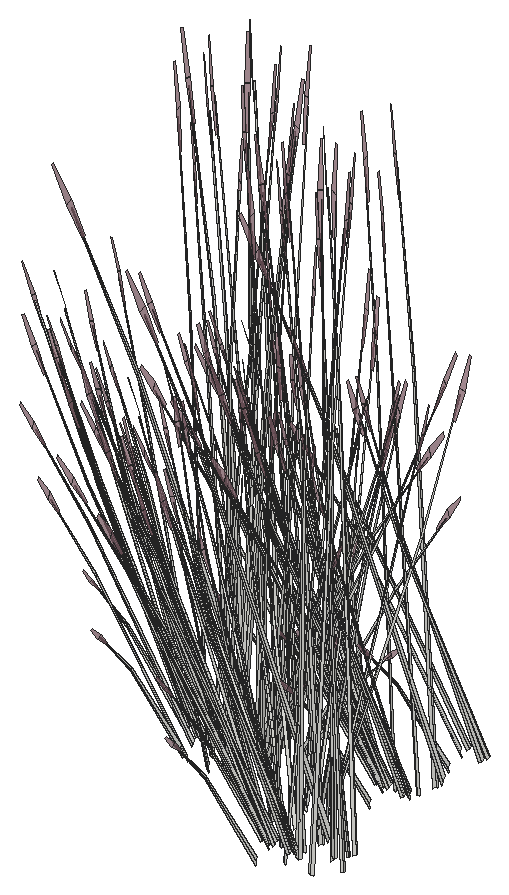
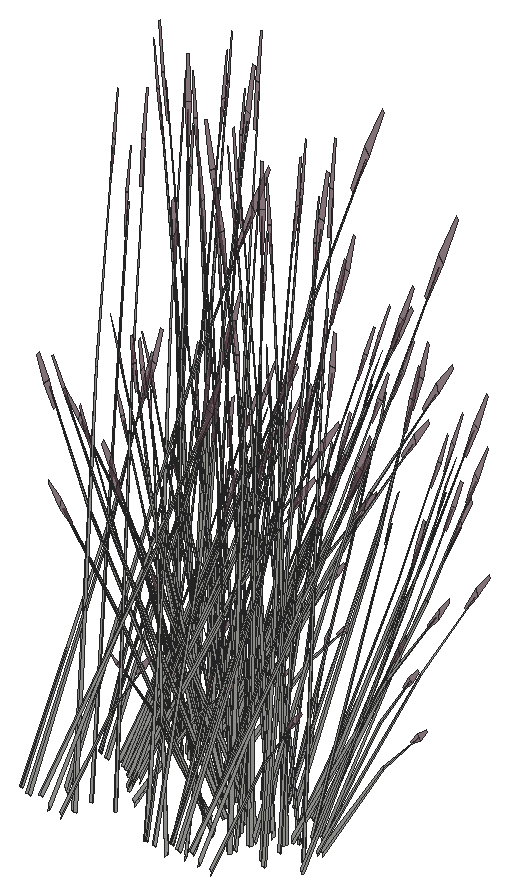
# SketchUp Ruby script. Lengths in inches.
U = 1.inch
M = Sketchup.active_model
def pt(a) = Geom::Point3d.new(a.map { |v| v * U })
def face(e, loops, mat)
  f = e.add_face(loops[0].map { |a| pt(a) })
  loops[1..].each { |l| e.add_face(l.map { |a| pt(a) }).erase! }
  f.material = f.back_material = mat if mat
  f
end
# faces: each face lists its corners as indices into pts; further lists are holes
def faces(e, pts, list, mat = nil) = list.each { |f| face(e, (f[0].is_a?(Array) ? f : [f]).map { |l| l.map { |i| pts[i] } }, mat) }
# xy, xz, yz: faces in a plane at the given z, y or x. An outline is a flat list of corners, or four numbers for a rectangle; further outlines are holes
def ring(l) = l.size == 4 ? [[l[0], l[1]], [l[2], l[1]], [l[2], l[3]], [l[0], l[3]]] : l.each_slice(2).to_a
def flat(e, list, mat, &to3) = list.each { |f| face(e, (f[0].is_a?(Array) ? f : [f]).map { |l| ring(l).map { |u, v| to3.(u, v) } }, mat) }
def xy(e, z, list, mat = nil) = flat(e, list, mat) { |x, y| [x, y, z] }
def xz(e, y, list, mat = nil) = flat(e, list, mat) { |x, z| [x, y, z] }
def yz(e, x, list, mat = nil) = flat(e, list, mat) { |y, z| [x, y, z] }
def lines(e, pts, list) = list.each { |a, b| e.add_line(pt(pts[a]), pt(pts[b])) }
# prism: a flat outline (further loops are holes) pulled along v
def prism(e, loops, v, mat = nil)
  f = face(e, loops, mat); d = Geom::Vector3d.new(v.map { |x| x * U })
  f.pushpull(f.normal.samedirection?(d) ? d.length : -d.length)
end
def box(e, o, s, mat = nil) = prism(e, [[o, [o[0] + s[0], o[1], o[2]], [o[0] + s[0], o[1] + s[1], o[2]], [o[0], o[1] + s[1], o[2]]]], [0, 0, s[2]], mat)
def at(x, y, z, deg = 0) = Geom::Transformation.translation(pt([x, y, z])) * Geom::Transformation.rotation(ORIGIN, Z_AXIS, deg.degrees)
def axes(o, x, y, z) = Geom::Transformation.new([*x, 0, *y, 0, *z, 0, *pt(o).to_a, 1])
def part(name) = M.definitions.add(name)
# library, detail: a bought-in or finely detailed component or shape, given as its bounding box
def library(name, o, s) = part(name).tap { |d| box(d.entities, o, s) }
def detail(e, o, s) = box(e.add_group.entities, o, s)
def put(e, d, t, mat = nil) = e.add_instance(d, t).tap { |i| i.material = mat if mat }
def group(e, t, mat = nil) = e.add_group.tap { |g| g.transformation = t; g.material = mat if mat }.entities
root = M.entities
M.materials.add("LightPink_Translucent").color = [144, 107, 117]
M.materials["LightPink_Translucent"].alpha = 0.75
c1 = part("blade")
p = [[2.15,0.21,22],[0,0.17,0],[0.09,0.45,0],[2.18,0.31,22],[2.29,0.31,22],[0.38,0.45,0],
  [2.48,0.24,33],[2.49,0.24,33],[2.48,0.22,33]]
faces(c1.entities,p,[[0,1,2,3],[4,5,2,3],[6,3,4,7],[8,0,3,6]])
c2 = part("seeds")
p = [[0.3,-0.1,1.38],[-0.01,-0.03,1.59],[-0.01,-0.03,0.03],[0.14,-0.07,-0.07],[0.29,-0.03,3],[0.15,0.01,3.11]]
faces(c2.entities,p,[[0,1,2,3],[1,0,4,5]],"LightPink_Translucent")
c3 = part("blade with seeds")
put(c3.entities,c1,at(0,0,0))
put(c3.entities,c2,axes([2.4,0.25,30.99],[1.5799,-0.05474,1.17369],[-0.12525,1.92788,0.29478],[-0.07173,-0.02425,1.56792]))
put(root,c3,axes([675.71,330.72,513.22],[0.14872,0.18332,1.42242],[-0.6872,0.15433,0.11501],[-0.15531,-0.28779,0.60807]))
put(root,c3,axes([677.54,330.86,514.13],[-0.31051,-0.46426,-0.58968],[0.63919,-0.25873,0.07116],[-0.07261,-0.22432,0.83415]))
put(root,c3,axes([677.6,330.46,513.76],[0.19614,-0.43908,-0.29394],[0.57222,0.12807,0.37948],[-0.05247,-0.17678,0.72609]))
put(root,c3,axes([677.31,330.76,513.89],[-0.63954,-0.14313,-0.42412],[0.21921,-0.49074,-0.32852],[-0.05864,-0.19758,0.81151]))
put(root,c3,axes([675.33,329.93,512.3],[0.33937,0.19872,0.95334],[-0.49424,0.11946,0.70045],[-0.10575,-0.15273,0.20998]))
put(root,c3,axes([676.14,330.99,514.13],[-0.55475,-0.27598,-0.58968],[0.39425,-0.48361,0.07116],[-0.20099,-0.16478,0.83415]))
put(root,c3,axes([675.95,330.62,513.76],[-0.10048,-0.4599,-0.29394],[0.5744,-0.12144,0.37948],[-0.15428,-0.13179,0.72609]))
put(root,c3,axes([674.72,331.29,513.22],[0.24166,0.09837,1.42242],[-0.50011,0.41269,0.11501],[-0.3117,-0.18617,0.60807]))
put(root,c3,axes([675.88,331,513.89],[-0.64198,0.13573,-0.42412],[-0.1123,-0.514,-0.32852],[-0.17243,-0.1473,0.81151]))
put(root,c3,axes([677.47,334.11,512.76],[0.56221,0.23024,1.25546],[-0.55078,0.49601,0.49647],[-0.2467,-0.29398,1.05249]))
put(root,c3,axes([674.62,331.43,513.76],[-0.37017,-0.35748,-0.29394],[0.42268,-0.3384,0.37948],[-0.21476,-0.05149,0.72609]))
put(root,c3,axes([675.01,331.67,514.13],[-0.65035,-0.01375,-0.58968],[0.04368,-0.5789,0.07116],[-0.27552,-0.06109,0.83415]))
put(root,c3,axes([674.8,331.79,513.89],[-0.47241,0.37822,-0.42412],[-0.41372,-0.39954,-0.32852],[-0.24002,-0.05755,0.81151]))
put(root,c3,axes([673.73,332.29,512.3],[0.41536,-0.04086,0.95334],[-0.26347,0.35999,0.70045],[-0.20525,-0.054,0.20998]))
put(root,c3,axes([676.67,332.62,512.26],[-0.70648,0.03525,0.37133],[-0.06389,-0.58508,-0.17871],[0.12647,-0.0593,1.19224]))
put(root,c3,axes([674.84,333.05,512.06],[0,0.57097,0.4121],[-0.72788,0,0],[0,-0.13004,1.30728]))
put(root,c3,axes([674.21,332.19,513.22],[0.26985,-0.01293,1.42242],[-0.17902,0.56047,0.11501],[-0.38456,-0.03467,0.60807]))
put(root,c3,axes([676.5,333.34,512.26],[-0.31565,0.51449,0.37133],[-0.65588,-0.24761,-0.17871],[0,-0.1186,1.19224]))
put(root,c3,axes([676.34,331.62,512.05],[-0.18794,0.56744,0.14643],[-0.68774,-0.16058,0.29122],[0.1188,-0.00276,1.33138]))
put(root,c3,axes([676.27,334.54,512.05],[0.6991,-0.15154,0.14643],[0.17263,0.56398,0.29122],[-0.06235,-0.08217,1.33138]))
put(root,c3,axes([673.97,332.67,513.76],[-0.54068,-0.15928,-0.29394],[0.1577,-0.46469,0.37948],[-0.21769,0.04261,0.72609]))
put(root,c3,axes([678.42,331.65,512.05],[-0.6991,0.15154,0.14643],[-0.17263,-0.56398,0.29122],[0.06235,0.08217,1.33138]))
put(root,c3,axes([666.76,337.92,512.15],[-0.18493,0.11557,1.18691],[-0.55384,-0.20228,-0.25526],[0.10266,-0.25157,0.50747]))
put(root,c3,axes([665.92,338.32,514.13],[-0.31051,-0.46426,-0.58968],[0.63919,-0.25873,0.07116],[-0.07261,-0.22432,0.83415]))
put(root,c3,axes([663.9,337.7,512.15],[-0.0394,0.18678,1.18691],[-0.57594,0.15636,-0.25526],[-0.13463,-0.24142,0.50747]))
put(root,c3,axes([678.35,334.57,512.05],[0.18794,-0.56744,0.14643],[0.68774,0.16058,0.29122],[-0.1188,0.00276,1.33138]))
put(root,c3,axes([667.21,338.77,514.13],[0.01693,-0.52814,-0.58968],[0.71285,0.03547,0.07116],[0.07523,-0.22375,0.83415]))
put(root,c3,axes([675.62,332.59,512.77],[0.18493,-0.0826,1.46963],[0.06377,0.5767,0.11501],[-0.40056,0.07652,0.52526]))
put(root,c3,axes([679.43,333.125,512.05],[-0.51116,-0.4159,0.14643],[0.51512,-0.4034,0.29122],[-0.05645,0.08494,1.33138]))
put(root,c3,axes([665.98,337.93,513.76],[0.19614,-0.43908,-0.29394],[0.57222,0.12807,0.37948],[-0.05247,-0.17678,0.72609]))
put(root,c3,axes([666.41,338.51,513.22],[-0.12114,0.19625,1.42242],[-0.50818,-0.40613,0.11501],[0.22925,-0.25313,0.60807]))
put(root,c3,axes([676.04,334.83,512.06],[0.60889,0.28548,0.4121],[-0.36394,0.51192,0],[-0.13868,-0.06502,1.30728]))
put(root,c3,axes([665.68,338.23,513.89],[-0.63954,-0.14313,-0.42412],[0.21921,-0.49074,-0.32852],[-0.05864,-0.19758,0.81151]))
put(root,c3,axes([666.08,337,512.3],[0.08346,0.33295,0.95334],[-0.46298,-0.1844,0.70045],[0.04982,-0.17048,0.20998]))
put(root,c3,axes([667.07,338.6,513.89],[-0.46573,-0.38364,-0.42412],[0.49199,-0.33598,-0.32852],[0.07086,-0.19492,0.81151]))
put(root,c3,axes([674.34,332.91,513.89],[-0.17625,0.51936,-0.42412],[-0.60429,-0.17802,-0.32852],[-0.2433,0.04762,0.81151]))
put(root,c3,axes([678.02,333.57,512.26],[0.70648,-0.03525,0.37133],[0.06389,0.58508,-0.17871],[-0.12647,0.0593,1.19224]))
put(root,c3,axes([667.5,338.46,513.76],[0.4402,-0.30062,-0.29394],[0.41671,0.34326,0.37948],[0.0634,-0.1744,0.72609]))
put(root,c3,axes([663.7,337.4,512.3],[0.33937,0.19872,0.95334],[-0.49424,0.11946,0.70045],[-0.10575,-0.15273,0.20998]))
put(root,c3,axes([664.52,338.45,514.13],[-0.55475,-0.27598,-0.58968],[0.39425,-0.48361,0.07116],[-0.20099,-0.16478,0.83415]))
put(root,c3,axes([664.33,338.09,513.76],[-0.10048,-0.4599,-0.29394],[0.5744,-0.12144,0.37948],[-0.15428,-0.13179,0.72609]))
put(root,c3,axes([674.32,333.18,513.22],[0.22574,-0.12077,1.42242],[0.19004,0.55807,0.11501],[-0.35439,0.12613,0.60807]))
put(root,c3,axes([676.7,340.4,513.22],[0.14872,0.18332,1.42242],[-0.6872,0.15433,0.11501],[-0.15531,-0.28779,0.60807]))
put(root,c3,axes([678.53,340.53,514.13],[-0.31051,-0.46426,-0.58968],[0.63919,-0.25873,0.07116],[-0.07261,-0.22432,0.83415]))
put(root,c3,axes([678.55,334.88,512.06],[0.60889,-0.28548,0.4121],[0.36394,0.51192,0],[-0.13868,0.06502,1.30728]))
put(root,c3,axes([664.26,338.47,513.89],[-0.64198,0.13573,-0.42412],[-0.1123,-0.514,-0.32852],[-0.17243,-0.1473,0.81151]))
put(root,c3,axes([668.05,339.69,514.13],[0.33983,-0.45051,-0.58968],[0.59551,0.32017,0.07116],[0.20291,-0.16322,0.83415]))
put(root,c3,axes([673.14,335.13,512.3],[0.27113,-0.25877,0.95334],[0.10699,0.40966,0.70045],[-0.19594,0.07335,0.20998]))
put(root,c3,axes([668.03,339.48,513.89],[-0.16713,-0.52135,-0.42412],[0.63294,-0.0912,-0.32852],[0.18138,-0.14003,0.81151]))
put(root,c3,axes([674.17,334.01,513.76],[-0.56631,0.0816,-0.29394],[-0.14954,-0.46647,0.37948],[-0.16229,0.12529,0.72609]))
put(root,c3,axes([678.59,340.14,513.76],[0.19614,-0.43908,-0.29394],[0.57222,0.12807,0.37948],[-0.05247,-0.17678,0.72609]))
put(root,c3,axes([678.3,340.4375,513.89],[-0.63954,-0.14313,-0.42412],[0.21921,-0.49074,-0.32852],[-0.05864,-0.19758,0.81151]))
put(root,c3,axes([665.85,341.57,512.76],[0.56221,0.23024,1.25546],[-0.55078,0.49601,0.49647],[-0.2467,-0.29398,1.05249]))
put(root,c3,axes([668.54,339.28,512.15],[-0.23242,-0.01691,1.18691],[-0.23811,-0.45367,-0.25526],[0.28553,-0.12834,0.50747]))
put(root,c3,axes([668.81,338.44,512.3],[-0.2167,0.29065,0.95334],[-0.18626,-0.3905,0.70045],[0.17898,-0.09785,0.20998]))
put(root,c3,axes([676.3125,339.61,512.3],[0.33937,0.19872,0.95334],[-0.49424,0.11946,0.70045],[-0.10575,-0.15273,0.20998]))
put(root,c3,axes([677.13,340.66,514.13],[-0.55475,-0.27598,-0.58968],[0.39425,-0.48361,0.07116],[-0.20099,-0.16478,0.83415]))
put(root,c3,axes([676.94,340.3,513.76],[-0.10048,-0.4599,-0.29394],[0.5744,-0.12144,0.37948],[-0.15428,-0.13179,0.72609]))
put(root,c3,axes([668.5,339.54,513.76],[0.56631,-0.0816,-0.29394],[0.14954,0.46647,0.37948],[0.16229,-0.12529,0.72609]))
put(root,c3,axes([675.14,333.55,513.22],[0.1625,-0.17544,1.42242],[0.41029,0.47354,0.11501],[-0.28141,0.21565,0.60807]))
put(root,c3,axes([674.63,334.07,513.89],[0.16713,0.52135,-0.42412],[-0.63294,0.0912,-0.32852],[-0.18138,0.14003,0.81151]))
put(root,c3,axes([663,338.9,513.76],[-0.37017,-0.35748,-0.29394],[0.42268,-0.3384,0.37948],[-0.21476,-0.05149,0.72609]))
put(root,c3,axes([678.34,333.01,512.36],[-0.01777,-0.53759,1.17256],[0.80434,0.13935,0.49647],[-0.19024,0.29416,1.1068]))
put(root,c3,axes([662.86,339.27,512.15],[0.12702,0.15896,1.18691],[-0.2927,0.4321,-0.25526],[-0.30054,-0.10328,0.50747]))
put(root,c3,axes([675.7,340.97,513.22],[0.24166,0.09837,1.42242],[-0.50011,0.41269,0.11501],[-0.3117,-0.18617,0.60807]))
put(root,c3,axes([663.39,339.13,514.13],[-0.65035,-0.01375,-0.58968],[0.04368,-0.5789,0.07116],[-0.27552,-0.06109,0.83415]))
put(root,c3,axes([676.875,340.68,513.89],[-0.64198,0.13573,-0.42412],[-0.1123,-0.514,-0.32852],[-0.17243,-0.1473,0.81151]))
put(root,c3,axes([675.02,333.99,513.22],[0.12114,-0.19625,1.42242],[0.50818,0.40613,0.11501],[-0.22925,0.25313,0.60807]))
put(root,c3,axes([675.16,335.09,513.76],[-0.4402,0.30062,-0.29394],[-0.41671,-0.34326,0.37948],[-0.0634,0.1744,0.72609]))
put(root,c3,axes([663.17,339.25,513.89],[-0.47241,0.37822,-0.42412],[-0.41372,-0.39954,-0.32852],[-0.24002,-0.05755,0.81151]))
put(root,c3,axes([675.44,336.26,512.3],[-0.01684,-0.3395,0.95334],[0.42072,0.24214,0.70045],[-0.08274,0.16182,0.20998]))
put(root,c3,axes([662.11,339.75,512.3],[0.41536,-0.04086,0.95334],[-0.26347,0.35999,0.70045],[-0.20525,-0.054,0.20998]))
put(root,c3,axes([678.46,343.79,512.76],[0.56221,0.23024,1.25546],[-0.55078,0.49601,0.49647],[-0.2467,-0.29398,1.05249]))
put(root,c3,axes([665.04,340.09,512.26],[-0.70648,0.03525,0.37133],[-0.06389,-0.58508,-0.17871],[0.12647,-0.0593,1.19224]))
put(root,c3,axes([663.22,340.51,512.06],[0,0.57097,0.4121],[-0.72788,0,0],[0,-0.13004,1.30728]))
put(root,c3,axes([668.33,340.64,513.89],[0.17625,-0.51936,-0.42412],[0.60429,0.17802,-0.32852],[0.2433,-0.04762,0.81151]))
put(root,c3,axes([675.6,334.95,514.15],[0.46573,0.38364,-0.47077],[-0.49199,0.33598,-0.36465],[-0.07086,0.19492,0.90078]))
put(root,c3,axes([664.875,340.8,512.26],[-0.31565,0.51449,0.37133],[-0.65588,-0.24761,-0.17871],[0,-0.1186,1.19224]))
put(root,c3,axes([676.69,335.62,513.76],[-0.19614,0.43908,-0.29394],[-0.57222,-0.12807,0.37948],[0.05247,0.17678,0.72609]))
put(root,c3,axes([667.02,338.82,512.06],[-0.60889,-0.28548,0.4121],[0.36394,-0.51192,0],[0.13868,0.06502,1.30728]))
put(root,c3,axes([668.21,340.83,514.13],[0.57168,-0.25217,-0.58968],[0.3186,0.51908,0.07116],[0.27622,-0.05897,0.83415]))
put(root,c3,axes([675.46,334.77,514.43],[-0.01693,0.52814,-0.65454],[-0.71285,-0.03547,0.07899],[-0.07523,0.22375,0.92591]))
put(root,c3,axes([675.61,341.11,513.76],[-0.37017,-0.35748,-0.29394],[0.42268,-0.3384,0.37948],[-0.21476,-0.05149,0.72609]))
put(root,c3,axes([676.13,334.4,513.22],[-0.01592,-0.21915,1.42242],[0.69015,0.14538,0.11501],[-0.04269,0.3123,0.60807]))
put(root,c3,axes([664.71,339.08,512.05],[-0.18794,0.56744,0.14643],[-0.68774,-0.16058,0.29122],[0.1188,-0.00276,1.33138]))
put(root,c3,axes([676.75,335.23,514.13],[0.31051,0.46426,-0.58968],[-0.63919,0.25873,0.07116],[0.07261,0.22432,0.83415]))
put(root,c3,axes([676,341.35,514.13],[-0.65035,-0.01375,-0.58968],[0.04368,-0.5789,0.07116],[-0.27552,-0.06109,0.83415]))
put(root,c3,axes([665.89,339.85,512.26],[-0.39083,-0.47924,0.37133],[0.59199,-0.33747,-0.17871],[0.12647,0.0593,1.19224]))
put(root,c3,axes([664.65,342.01,512.05],[0.6991,-0.15154,0.14643],[0.17263,0.56398,0.29122],[-0.06235,-0.08217,1.33138]))
put(root,c3,axes([668.7,340.875,513.76],[0.54068,0.15928,-0.29394],[-0.1577,0.46469,0.37948],[0.21769,-0.04261,0.72609]))
put(root,c3,axes([662.34,340.14,513.76],[-0.54068,-0.15928,-0.29394],[0.1577,-0.46469,0.37948],[-0.21769,0.04261,0.72609]))
put(root,c3,axes([666.79,339.11,512.05],[-0.6991,0.15154,0.14643],[-0.17263,-0.56398,0.29122],[0.06235,0.08217,1.33138]))
put(root,c3,axes([675.22,335.52,512.79],[0.01429,-0.29475,1.28107],[0.64291,0.15569,0.17703],[-0.0557,0.31414,0.60492]))
put(root,c3,axes([667.22,340.3,513.22],[-0.26985,0.01293,1.42242],[0.17902,-0.56047,0.11501],[0.38456,0.03467,0.60807]))
put(root,c3,axes([675.79,341.46,513.89],[-0.47241,0.37822,-0.42412],[-0.41372,-0.39954,-0.32852],[-0.24002,-0.05755,0.81151]))
put(root,c3,axes([674.72,341.96,512.3],[0.41536,-0.04086,0.95334],[-0.26347,0.35999,0.70045],[-0.20525,-0.054,0.20998]))
put(root,c3,axes([675.83,342.72,512.06],[0,0.57097,0.4121],[-0.72788,0,0],[0,-0.13004,1.30728]))
put(root,c3,axes([666.73,342.04,512.05],[0.18794,-0.56744,0.14643],[0.68774,0.16058,0.29122],[-0.1188,0.00276,1.33138]))
put(root,c3,axes([675.19,341.87,513.22],[0.26985,-0.01293,1.42242],[-0.17902,0.56047,0.11501],[-0.38456,-0.03467,0.60807]))
put(root,c3,axes([663.99,340.06,512.77],[0.18493,-0.0826,1.46963],[0.06377,0.5767,0.11501],[-0.40056,0.07652,0.52526]))
put(root,c3,axes([667.8,340.59,512.05],[-0.51116,-0.4159,0.14643],[0.51512,-0.4034,0.29122],[-0.05645,0.08494,1.33138]))
put(root,c3,axes([669.84,340.97,512.3],[-0.40197,0.09426,0.95334],[0.18921,-0.38956,0.70045],[0.21325,0.02666,0.20998]))
put(root,c3,axes([677.49,343.01,512.26],[-0.31565,0.51449,0.37133],[-0.65588,-0.24761,-0.17871],[0,-0.1186,1.19224]))
put(root,c3,axes([666.34,346.52,513.22],[0.14872,0.18332,1.42242],[-0.6872,0.15433,0.11501],[-0.15531,-0.28779,0.60807]))
put(root,c3,axes([664.42,342.3,512.06],[0.60889,0.28548,0.4121],[-0.36394,0.51192,0],[-0.13868,-0.06502,1.30728]))
put(root,c3,axes([666.5625,340.32,512.26],[0.31565,-0.51449,0.37133],[0.65588,0.24761,-0.17871],[0,0.1186,1.19224]))
put(root,c3,axes([677.65,346.73,513.22],[0.14872,0.18332,1.42242],[-0.6872,0.15433,0.11501],[-0.15531,-0.28779,0.60807]))
put(root,c3,axes([668.17,346.66,514.13],[-0.31051,-0.46426,-0.58968],[0.63919,-0.25873,0.07116],[-0.07261,-0.22432,0.83415]))
put(root,c3,axes([662.71,340.375,513.89],[-0.17625,0.51936,-0.42412],[-0.60429,-0.17802,-0.32852],[-0.2433,0.04762,0.81151]))
put(root,c3,axes([669.15,342.17,513.26],[-0.12452,-0.47997,-0.02898],[0.58854,-0.11034,-0.1314],[0.1229,0.03043,0.43341]))
put(root,c3,axes([679.48,346.86,514.13],[-0.31051,-0.46426,-0.58968],[0.63919,-0.25873,0.07116],[-0.07261,-0.22432,0.83415]))
put(root,c3,axes([668.22,340.61,512.06],[0,-0.57097,0.4121],[0.72788,0,0],[0,0.13004,1.30728]))
put(root,c3,axes([666.4,341.03,512.26],[0.70648,-0.03525,0.37133],[0.06389,0.58508,-0.17871],[-0.12647,0.0593,1.19224]))
put(root,c3,axes([669.47,347.12,514.13],[0.01693,-0.52814,-0.58968],[0.71285,0.03547,0.07116],[0.07523,-0.22375,0.83415]))
put(root,c3,axes([669.09,341.6,512.15],[-0.15668,-0.14043,1.18691],[0.20386,-0.46454,-0.25526],[0.31701,0.06293,0.50747]))
put(root,c3,axes([668.23,346.27,513.76],[0.19614,-0.43908,-0.29394],[0.57222,0.12807,0.37948],[-0.05247,-0.17678,0.72609]))
put(root,c3,axes([668.66,346.85,513.22],[-0.12114,0.19625,1.42242],[-0.50818,-0.40613,0.11501],[0.22925,-0.25313,0.60807]))
put(root,c3,axes([677.26,344.22,512.05],[0.6991,-0.15154,0.14643],[0.17263,0.56398,0.29122],[-0.06235,-0.08217,1.33138]))
put(root,c3,axes([667.94,346.57,513.89],[-0.63954,-0.14313,-0.42412],[0.21921,-0.49074,-0.32852],[-0.05864,-0.19758,0.81151]))
put(root,c3,axes([668.34,345.34,512.3],[0.08346,0.33295,0.95334],[-0.46298,-0.1844,0.70045],[0.04982,-0.17048,0.20998]))
put(root,c3,axes([669.32,346.94,513.89],[-0.46573,-0.38364,-0.42412],[0.49199,-0.33598,-0.32852],[0.07086,-0.19492,0.81151]))
put(root,c3,axes([674.96,342.35,513.76],[-0.54068,-0.15928,-0.29394],[0.1577,-0.46469,0.37948],[-0.21769,0.04261,0.72609]))
put(root,c3,axes([679.25,346.77,513.89],[-0.63954,-0.14313,-0.42412],[0.21921,-0.49074,-0.32852],[-0.05864,-0.19758,0.81151]))
put(root,c3,axes([667.65,341.88,514.13],[0.65035,0.01375,-0.58968],[-0.04368,0.5789,0.07116],[0.27552,0.06109,0.83415]))
put(root,c3,axes([666.92,342.34,512.06],[0.60889,-0.28548,0.4121],[0.36394,0.51192,0],[-0.13868,0.06502,1.30728]))
put(root,c3,axes([669.76,346.8,513.76],[0.4402,-0.30062,-0.29394],[0.41671,0.34326,0.37948],[0.0634,-0.1744,0.72609]))
put(root,c3,axes([665.96,345.74,512.3],[0.33937,0.19872,0.95334],[-0.49424,0.11946,0.70045],[-0.10575,-0.15273,0.20998]))
put(root,c3,axes([666.77,346.79,514.13],[-0.55475,-0.27598,-0.58968],[0.39425,-0.48361,0.07116],[-0.20099,-0.16478,0.83415]))
put(root,c3,axes([666.58,346.43,513.76],[-0.10048,-0.4599,-0.29394],[0.5744,-0.12144,0.37948],[-0.15428,-0.13179,0.72609]))
put(root,c3,axes([661.99,341.59,512.15],[0.2261,0.04687,1.18691],[0.14573,0.47875,-0.25526],[-0.30712,0.08962,0.50747]))
put(root,c3,axes([677.26,345.94,512.3],[0.33937,0.19872,0.95334],[-0.49424,0.11946,0.70045],[-0.10575,-0.15273,0.20998]))
put(root,c3,axes([678.08,347,514.13],[-0.55475,-0.27598,-0.58968],[0.39425,-0.48361,0.07116],[-0.20099,-0.16478,0.83415]))
